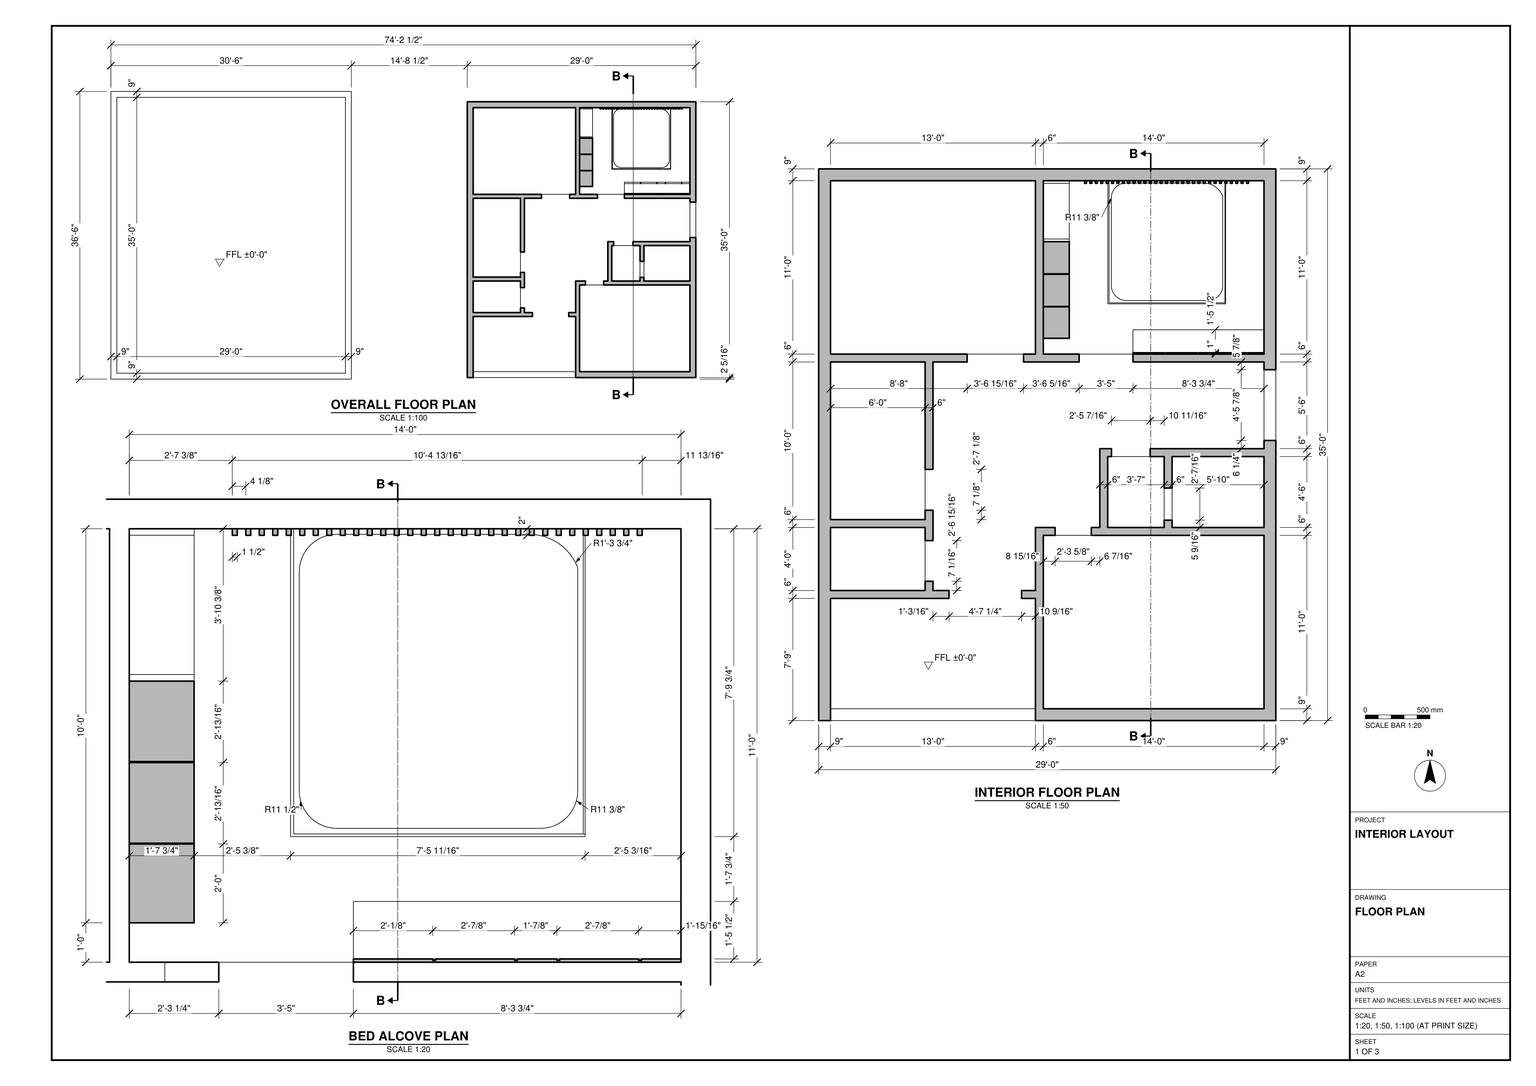
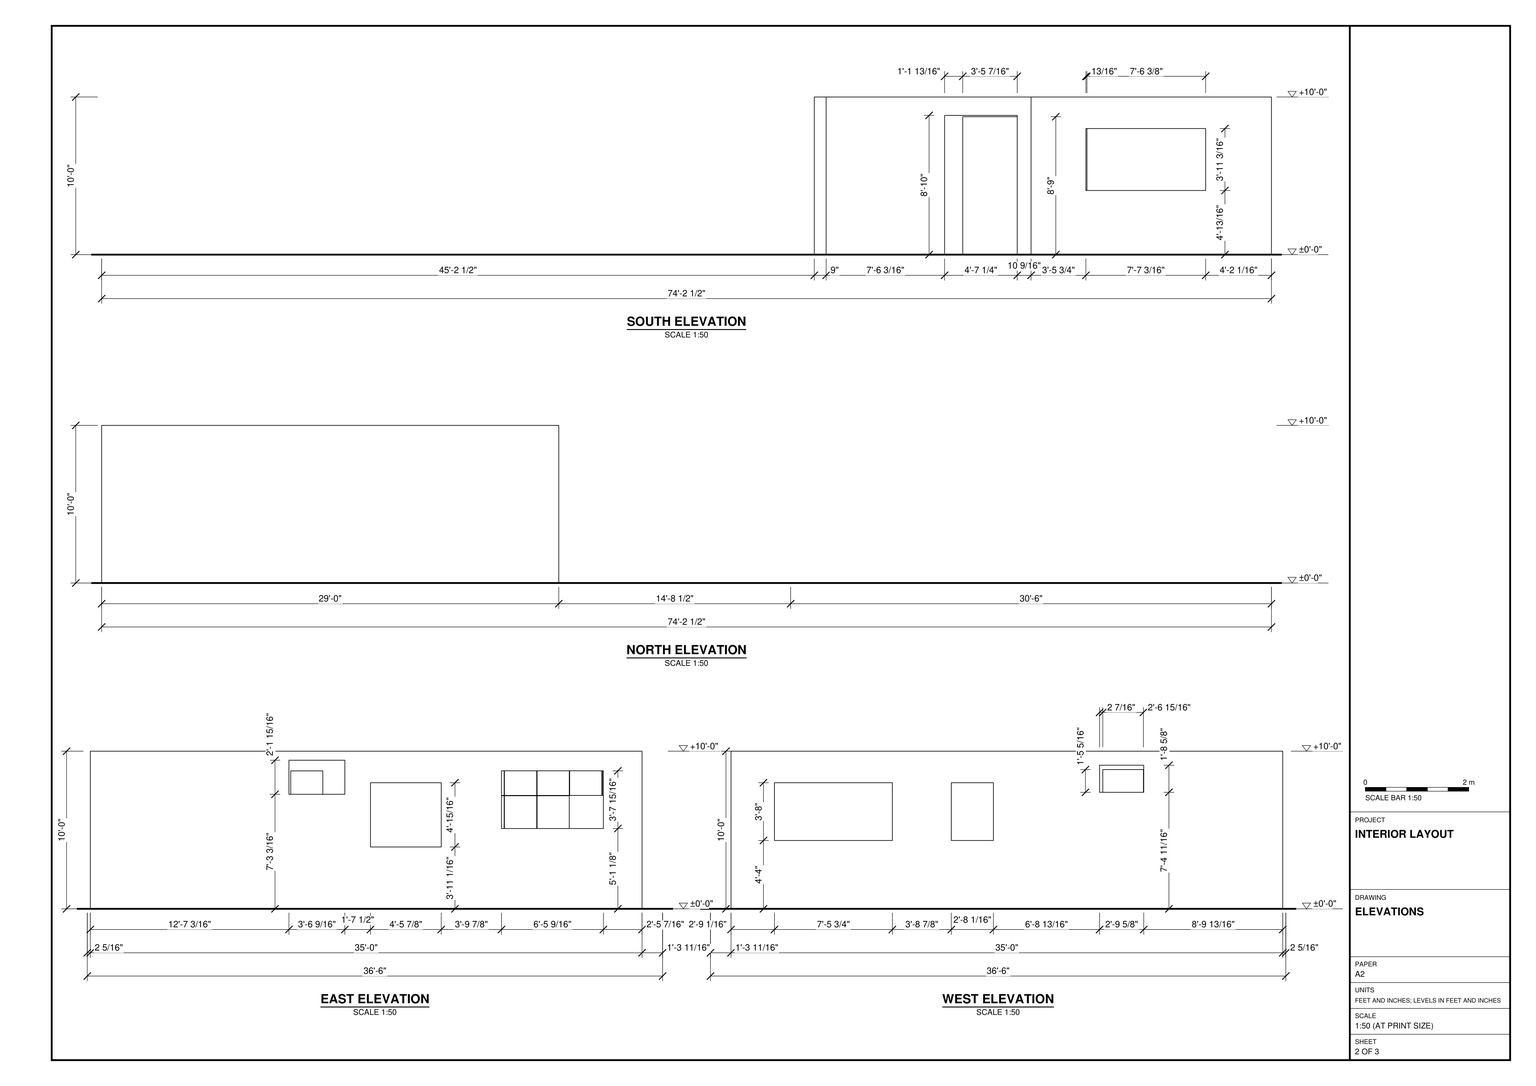
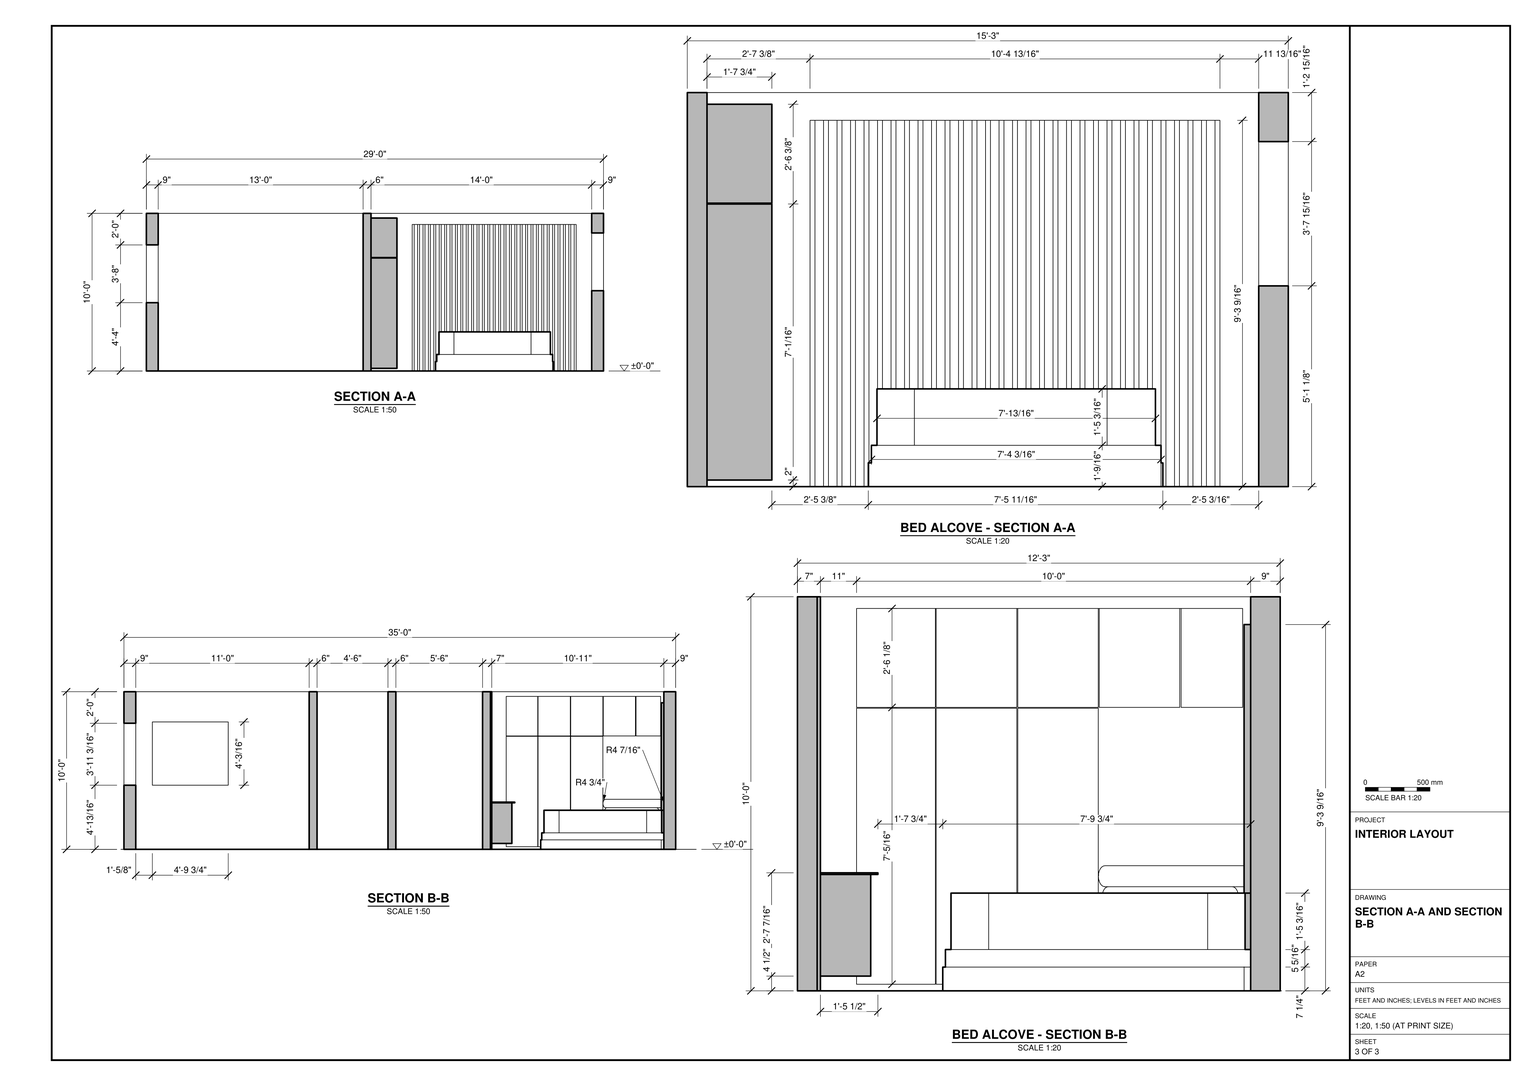
Work in feet and inches from task_files/diagram_01.pdf. Set the finished floor at ±0'-0". The full layout spans 74'-2 1/2" east to west, 36'-6" north to south and 10'-0" in height. Use the overall floor plan to place the flat, bordered rectangle on the west and the walled interior on the east. Leave the 14'-8 1/2" gap between them and follow the north and south offsets shown in plan.

Model the floor surfaces, exterior walls and partitions at their drawn thicknesses. Use the enlarged interior plan to set out the rooms and preserve the passages between them. Use the elevations to locate the south entrance and the window openings at their respective sill and head heights.

Fit out the northeast bed alcove using its enlarged plan and both sections. Model the stepped bed platform, the rounded mattress, the vertical slats behind the bed, the tall storage along the side wall and the shallow unit opposite the bed. Keep the entry beside the shallow unit clear. Make the shell elements and each furniture or joinery piece separate groups or components, and use components for repeated parts such as the slats. Any decor or loose items may be suitable library components. Save one SketchUp model as output_files/single_storey_interior_and_fitted_bed_alcove.skp.

# SketchUp Ruby script. Lengths in inches.
U = 1.inch
M = Sketchup.active_model
def pt(a) = Geom::Point3d.new(a.map { |v| v * U })
def face(e, loops, mat)
  f = e.add_face(loops[0].map { |a| pt(a) })
  loops[1..].each { |l| e.add_face(l.map { |a| pt(a) }).erase! }
  f.material = f.back_material = mat if mat
  f
end
# faces: each face lists its corners as indices into pts; further lists are holes
def faces(e, pts, list, mat = nil) = list.each { |f| face(e, (f[0].is_a?(Array) ? f : [f]).map { |l| l.map { |i| pts[i] } }, mat) }
# xy, xz, yz: faces in a plane at the given z, y or x. An outline is a flat list of corners, or four numbers for a rectangle; further outlines are holes
def ring(l) = l.size == 4 ? [[l[0], l[1]], [l[2], l[1]], [l[2], l[3]], [l[0], l[3]]] : l.each_slice(2).to_a
def flat(e, list, mat, &to3) = list.each { |f| face(e, (f[0].is_a?(Array) ? f : [f]).map { |l| ring(l).map { |u, v| to3.(u, v) } }, mat) }
def xy(e, z, list, mat = nil) = flat(e, list, mat) { |x, y| [x, y, z] }
def xz(e, y, list, mat = nil) = flat(e, list, mat) { |x, z| [x, y, z] }
def yz(e, x, list, mat = nil) = flat(e, list, mat) { |y, z| [x, y, z] }
def lines(e, pts, list) = list.each { |a, b| e.add_line(pt(pts[a]), pt(pts[b])) }
# prism: a flat outline (further loops are holes) pulled along v
def prism(e, loops, v, mat = nil)
  f = face(e, loops, mat); d = Geom::Vector3d.new(v.map { |x| x * U })
  f.pushpull(f.normal.samedirection?(d) ? d.length : -d.length)
end
def box(e, o, s, mat = nil) = prism(e, [[o, [o[0] + s[0], o[1], o[2]], [o[0] + s[0], o[1] + s[1], o[2]], [o[0], o[1] + s[1], o[2]]]], [0, 0, s[2]], mat)
def at(x, y, z, deg = 0) = Geom::Transformation.translation(pt([x, y, z])) * Geom::Transformation.rotation(ORIGIN, Z_AXIS, deg.degrees)
def axes(o, x, y, z) = Geom::Transformation.new([*x, 0, *y, 0, *z, 0, *pt(o).to_a, 1])
def part(name) = M.definitions.add(name)
# library, detail: a bought-in or finely detailed component or shape, given as its bounding box
def library(name, o, s) = part(name).tap { |d| box(d.entities, o, s) }
def detail(e, o, s) = box(e.add_group.entities, o, s)
def put(e, d, t, mat = nil) = e.add_instance(d, t).tap { |i| i.material = mat if mat }
def group(e, t, mat = nil) = e.add_group.tap { |g| g.transformation = t; g.material = mat if mat }.entities
root = M.entities
M.materials.add("[0099_LightSteelBlue]").color = [176, 196, 222]
M.materials.add("[Carrera Marble]").color = [207, 207, 207]
M.materials.add("[Color C07]").color = [153, 76, 0]
M.materials.add("[Color D06]").color = [204, 153, 0]
M.materials.add("[Suede Green]").color = [125, 126, 95]
M.materials.add("[Tile Canvas]").color = [199, 192, 173]
M.materials.add("[Wallpaper Thin Brown Stripes]").color = [182, 160, 118]
M.materials.add("[Wood Veneer 02]").color = [190, 128, 91]
xy(root,0,[[[0,0,366,438],[9,9,357,429]],[9,9,357,429],[551.52,11.34,707.52,11.34,707.52,95.34,699.55,95.34,699.55,101.34,707.52,101.34,707.52,149.34,722.48,149.34,722.48,143.34,750.09,143.34,750.09,149.34,756.52,149.34,756.52,209.34,765.4,209.34,765.4,203.34,794.85,203.34,794.85,209.34,881.52,209.34,881.52,275.34,781.77,275.34,781.77,281.34,724.34,281.34,724.34,275.34,698.46,275.34,698.46,281.34,655.52,281.34,655.52,275.34,629.52,275.34,629.52,193.59,623.52,193.59,623.52,162.46,629.52,162.46,629.52,139.34,623.52,139.34,623.52,108.4,629.52,108.4,629.52,101.34,641.71,101.34,641.71,95.34,551.52,95.34],[781.77,281.34,805.92,282.34],[805.92,281.34,806.82,281.9],
  [806.82,281.34,830.82,282.34],[830.82,281.34,831.72,281.9],[831.72,281.34,843.72,282.34],[843.72,281.34,844.625,281.9],[844.625,281.34,868.6,282.34],
  [868.6,281.34,869.53,281.9],[869.53,281.34,881.52,282.34],[744.9,411.34,746.4,413.34],[749.01,411.34,750.51,413.34],[753.12,411.34,754.62,413.34],
  [757.23,411.34,758.73,413.34],[855.88,411.34,857.38,413.34],[859.99,411.34,861.49,413.34],[864.1,411.34,865.6,413.34],[868.21,411.34,869.71,413.34]])
xy(root,0,[[762.65,319.59,762.65,411.34,762.84,411.34,762.84,413.34,851.77,413.34,851.77,411.34,852.33,411.34,852.33,319.59],[761.34,411.34,762.65,413.34],[762.65,411.34,762.84,413.34],[851.77,411.34,853.27,413.34]],"[Suede Green]")
xy(root,7.23,[[762.65,319.59,852.33,319.59,852.33,320.4,763.58,320.4,763.58,413.34,762.65,413.34],[851.77,320.4,852.33,411.34]],"[Suede Green]")
xy(root,12.57,[[[763.58,320.4,851.77,320.4,851.77,413.34,849.16,413.34,849.16,411.34,847.66,411.34,847.66,413.34,845.05,413.34,845.05,411.34,843.55,411.34,843.55,413.34,771.0625,413.34,771.0625,411.34,769.5625,411.34,769.5625,413.34,766.95,413.34,766.95,411.34,765.45,411.34,765.45,413.34,763.58,413.34],[776.75,322.1,775.25,322.2,773.78,322.49,772.36,322.97,771.02,323.63,769.77,324.47,768.64,325.46,767.65,326.59,766.82,327.83,766.15,329.18,765.67,330.6,765.38,332.07,765.28,333.57,765.28,400.26,765.375,401.74,765.67,403.2,766.15,404.61,766.8,405.95,767.63,407.1875,768.61,408.31,769.73,409.29,770.97,410.12,772.31,410.78,773.72,411.25,775.18,411.55,776.67,411.64,835.35,411.64,836.93,411.5625,838.5,411.32,840.03,410.93,841.52,410.38,842.94,409.69,844.29,408.86,845.55,407.89,846.7,406.81,847.74,405.61,848.66,404.31,849.4375,402.93,850.07,401.48,850.07,333.46,849.98,331.98,849.6875,330.52,849.21,329.11,848.55,327.78,847.73,326.54,846.75,325.43,845.63,324.45,844.39,323.62,843.06,322.96,841.65,322.48,840.19,322.19,838.71,322.1]]],"[Suede Green]")
xy(root,29.76,[[839.4375,411.34,840.9375,413.34]])
xy(root,29.76,[[776.75,322.1,838.71,322.1,840.19,322.19,841.65,322.48,843.06,322.96,844.39,323.62,845.63,324.45,846.75,325.43,847.73,326.54,848.55,327.78,849.21,329.11,849.6875,330.52,849.98,331.98,850.07,333.46,850.07,401.48,849.4375,402.93,848.66,404.31,847.74,405.61,846.7,406.81,845.55,407.89,844.29,408.86,842.94,409.69,841.52,410.38,840.03,410.93,838.5,411.32,836.93,411.5625,836.83,411.57,836.83,411.34,835.33,411.34,835.33,411.64,832.72,411.64,832.72,411.34,831.22,411.34,831.22,411.64,828.61,411.64,828.61,411.34,827.11,411.34,827.11,411.64,824.5,411.64,824.5,411.34,823,411.34,823,411.64,820.39,411.64,820.39,411.34,818.89,411.34,818.89,411.64,816.28,411.64,816.28,411.34,814.78,411.34,814.78,411.64,812.17,411.64,812.17,411.34,810.67,411.34,810.67,411.64,808.05,411.64,808.05,411.34,806.55,411.34,806.55,411.64,803.94,411.64,803.94,411.34,802.44,411.34,802.44,411.64,799.83,411.64,799.83,411.34,798.33,411.34,798.33,411.64,795.72,411.64,795.72,411.34,794.22,411.34,794.22,411.64,791.61,411.64,791.61,411.34,790.11,411.34,790.11,411.64,787.5,411.64,787.5,411.34,786,411.34,786,411.64,783.39,411.64,783.39,411.34,781.89,411.34,781.89,411.64,779.28,411.64,779.28,411.34,777.78,411.34,777.78,411.64,776.67,411.64,775.18,411.55,775.17,411.54,775.17,411.34,774.14,411.34,773.72,411.25,772.31,410.78,770.97,410.12,769.73,409.29,768.61,408.31,767.63,407.1875,766.8,405.95,766.15,404.61,765.67,403.2,765.375,401.74,765.28,400.26,765.28,333.57,765.38,332.07,765.67,330.6,766.15,329.18,766.82,327.83,767.65,326.59,768.64,325.46,769.77,324.47,771.02,323.63,772.36,322.97,773.78,322.49,775.25,322.2],[773.67,411.34,774.14,411.34,775.17,411.54,775.17,413.34,773.67,413.34],[774.14,411.34,775.17,411.34,775.17,411.54],[777.78,411.34,779.28,411.64],[781.89,411.34,783.39,411.64],
  [786,411.34,787.5,411.64],[790.11,411.34,791.61,411.64],[794.22,411.34,795.72,411.64],[798.33,411.34,799.83,411.64],[802.44,411.34,803.94,411.64],
  [806.55,411.34,808.05,411.64],[810.67,411.34,812.17,411.64],[814.78,411.34,816.28,411.64],[818.89,411.34,820.39,411.64],[823,411.34,824.5,411.64],
  [827.11,411.34,828.61,411.64],[831.22,411.34,832.72,411.64],[835.33,411.34,836.83,411.34,836.83,411.57,835.35,411.64,835.33,411.64],[836.83,411.57,836.83,413.34,835.33,413.34,835.33,411.64,835.35,411.64],[777.78,411.64,779.28,413.34],
  [781.89,411.64,783.39,413.34],[786,411.64,787.5,413.34],[790.11,411.64,791.61,413.34],[794.22,411.64,795.72,413.34],[798.33,411.64,799.83,413.34],
  [802.44,411.64,803.94,413.34],[806.55,411.64,808.05,413.34],[810.67,411.64,812.17,413.34],[814.78,411.64,816.28,413.34],[818.89,411.64,820.39,413.34],
  [823,411.64,824.5,413.34],[827.11,411.64,828.61,413.34],[831.22,411.64,832.72,413.34]],"[Suede Green]")
xy(root,111.55,[[744.9,411.34,746.4,413.34],[749.01,411.34,750.51,413.34],[753.12,411.34,754.62,413.34],[757.23,411.34,758.73,413.34],[761.34,411.34,762.84,413.34],
  [765.45,411.34,766.95,413.34],[769.5625,411.34,771.0625,413.34],[773.67,411.34,775.17,413.34],[777.78,411.34,779.28,413.34],[781.89,411.34,783.39,413.34],
  [786,411.34,787.5,413.34],[790.11,411.34,791.61,413.34],[794.22,411.34,795.72,413.34],[798.33,411.34,799.83,413.34],[802.44,411.34,803.94,413.34],
  [806.55,411.34,808.05,413.34],[810.67,411.34,812.17,413.34],[814.78,411.34,816.28,413.34],[818.89,411.34,820.39,413.34],[823,411.34,824.5,413.34],
  [827.11,411.34,828.61,413.34],[831.22,411.34,832.72,413.34],[835.33,411.34,836.83,413.34],[839.4375,411.34,840.9375,413.34],[843.55,411.34,845.05,413.34],
  [847.66,411.34,849.16,413.34],[851.77,411.34,853.27,413.34],[855.88,411.34,857.38,413.34],[859.99,411.34,861.49,413.34],[864.1,411.34,865.6,413.34],
  [868.21,411.34,869.71,413.34]],"[Wood Veneer 02]")
xy(root,120,[[805.92,281.34,806.82,281.9],[830.82,281.34,831.72,281.9],[843.72,281.34,844.625,281.9],[868.6,281.34,869.53,281.9]],"[Color D06]")
xy(root,120,[[781.77,281.34,805.92,282.34],[806.82,281.34,830.82,282.34],[831.72,281.34,843.72,282.34],[844.625,281.34,868.6,282.34],[869.53,281.34,881.52,282.34]],"[Wallpaper Thin Brown Stripes]")
xz(root,281.9,[[805.92,0,806.82,120],[830.82,0,831.72,120],[843.72,0,844.625,120],[868.6,0,869.53,120]],"[Color D06]")
xz(root,282.34,[[781.77,0,805.92,4.49],[806.82,0,830.82,4.49],[831.72,0,843.72,4.49],[844.625,0,868.6,4.49],[869.53,0,881.52,4.49],
  [781.77,4.49,805.92,35.4375],[805.92,4.49,806.82,35.4375],[806.82,4.49,830.82,35.4375],[830.82,4.49,831.72,35.4375],[831.72,4.49,843.72,35.4375],
  [843.72,4.49,844.625,35.4375],[844.625,4.49,868.6,35.4375],[868.6,4.49,869.53,35.4375]])
xz(root,282.34,[[781.77,35.4375,805.92,120],[806.82,35.4375,830.82,120],[831.72,35.4375,843.72,120],[844.625,35.4375,868.6,120],[869.53,35.4375,881.52,120]],"[Wallpaper Thin Brown Stripes]")
xz(root,319.59,[[762.65,0,852.33,7.23]],"[Suede Green]")
xz(root,320.4,[[763.58,7.23,851.77,12.57]],"[Suede Green]")
xz(root,322.1,[[776.75,12.57,838.71,29.76]],"[Suede Green]")
xz(root,411.34,[[851.77,0,852.33,7.23]],"[Suede Green]")
xz(root,411.34,[[744.9,0,746.4,111.55],[749.01,0,750.51,111.55],[753.12,0,754.62,111.55],[757.23,0,758.73,111.55],[761.34,0,762.84,111.55],
  [852.33,0,853.27,0,853.27,111.55,851.77,111.55,851.77,7.23,852.33,7.23],[855.88,0,857.38,111.55],[859.99,0,861.49,111.55],[864.1,0,865.6,111.55],[868.21,0,869.71,111.55],
  [765.45,12.57,766.95,111.55],[769.5625,12.57,771.0625,111.55],[843.55,12.57,845.05,111.55],[847.66,12.57,849.16,111.55],[773.67,29.76,775.17,111.55],
  [777.78,29.76,779.28,111.55],[781.89,29.76,783.39,111.55],[786,29.76,787.5,111.55],[790.11,29.76,791.61,111.55],[794.22,29.76,795.72,111.55],
  [798.33,29.76,799.83,111.55],[802.44,29.76,803.94,111.55],[806.55,29.76,808.05,111.55],[810.67,29.76,812.17,111.55],[814.78,29.76,816.28,111.55],
  [818.89,29.76,820.39,111.55],[823,29.76,824.5,111.55],[827.11,29.76,828.61,111.55],[831.22,29.76,832.72,111.55],[835.33,29.76,836.83,111.55],
  [839.4375,29.76,840.9375,111.55]],"[Wood Veneer 02]")
xz(root,411.64,[[776.67,12.57,835.35,29.76]],"[Suede Green]")
xz(root,413.34,[[744.9,0,746.4,37.01],[749.01,0,750.51,111.55],[753.12,0,754.62,111.55],[757.23,0,758.73,111.55],[855.88,0,857.38,111.55],
  [859.99,0,861.49,111.55],[864.1,0,865.6,111.55],[868.21,0,869.52,111.55],[869.52,0,869.71,37.01],[839.4375,29.76,840.9375,111.55]])
xz(root,413.34,[[761.34,0,762.65,0,762.65,7.23,762.84,7.23,762.84,111.55,761.34,111.55],[762.65,0,762.84,7.23],[762.84,0,762.84,7.23,763.58,7.23,763.58,12.57,765.45,12.57,765.45,27.14,766.95,27.14,766.95,12.57,769.5625,12.57,769.5625,27.14,771.0625,27.14,771.0625,12.57,843.55,12.57,843.55,27.14,845.05,27.14,845.05,12.57,847.66,12.57,847.66,27.14,849.16,27.14,849.16,12.57,851.77,12.57,851.77,0],[851.77,0,853.27,111.55],[765.45,27.14,766.95,111.55],
  [769.5625,27.14,771.0625,111.55],[843.55,27.14,845.05,111.55],[847.66,27.14,849.16,111.55],[773.67,29.76,775.17,111.55],[777.78,29.76,779.28,111.55],
  [781.89,29.76,783.39,111.55],[786,29.76,787.5,111.55],[790.11,29.76,791.61,111.55],[794.22,29.76,795.72,111.55],[798.33,29.76,799.83,111.55],
  [802.44,29.76,803.94,111.55],[806.55,29.76,808.05,111.55],[810.67,29.76,812.17,111.55],[814.78,29.76,816.28,111.55],[818.89,29.76,820.39,111.55],
  [823,29.76,824.5,111.55],[827.11,29.76,828.61,111.55],[831.22,29.76,832.72,111.55],[835.33,29.76,836.83,111.55]],"[Suede Green]")
yz(root,744.9,[[411.34,0,413.34,111.55]],"[Wood Veneer 02]")
yz(root,746.4,[[411.34,0,413.34,111.55]],"[Wood Veneer 02]")
yz(root,749.01,[[411.34,0,413.34,111.55]],"[Wood Veneer 02]")
yz(root,750.51,[[411.34,0,413.34,111.55]],"[Wood Veneer 02]")
yz(root,753.12,[[411.34,0,413.34,111.55]],"[Wood Veneer 02]")
yz(root,754.62,[[411.34,0,413.34,111.55]],"[Wood Veneer 02]")
yz(root,757.23,[[411.34,0,413.34,111.55]],"[Wood Veneer 02]")
yz(root,758.73,[[411.34,0,413.34,111.55]],"[Wood Veneer 02]")
yz(root,761.34,[[411.34,0,413.34,111.55]],"[Wood Veneer 02]")
yz(root,762.65,[[319.59,0,413.34,7.23]],"[Suede Green]")
yz(root,762.84,[[411.34,0,413.34,111.55]],"[Wood Veneer 02]")
yz(root,763.58,[[320.4,7.23,413.34,12.57]],"[Suede Green]")
yz(root,765.28,[[333.57,12.57,400.26,29.76]],"[Suede Green]")
yz(root,765.45,[[411.34,12.57,413.34,111.55]],"[Wood Veneer 02]")
yz(root,766.95,[[411.34,12.57,413.34,111.55]],"[Wood Veneer 02]")
yz(root,769.5625,[[411.34,12.57,413.34,111.55]],"[Wood Veneer 02]")
yz(root,771.0625,[[411.34,12.57,413.34,111.55]],"[Wood Veneer 02]")
yz(root,773.67,[[411.34,29.76,413.34,111.55]],"[Wood Veneer 02]")
yz(root,775.17,[[411.34,29.76,413.34,111.55]],"[Wood Veneer 02]")
yz(root,777.78,[[411.34,29.76,413.34,111.55]],"[Wood Veneer 02]")
yz(root,779.28,[[411.34,29.76,413.34,111.55]],"[Wood Veneer 02]")
yz(root,781.77,[[281.34,0,282.34,120]],"[Color D06]")
yz(root,781.89,[[411.34,29.76,413.34,111.55]],"[Wood Veneer 02]")
yz(root,783.39,[[411.34,29.76,413.34,111.55]],"[Wood Veneer 02]")
yz(root,786,[[411.34,29.76,413.34,111.55]],"[Wood Veneer 02]")
yz(root,787.5,[[411.34,29.76,413.34,111.55]],"[Wood Veneer 02]")
yz(root,790.11,[[411.34,29.76,413.34,111.55]],"[Wood Veneer 02]")
yz(root,791.61,[[411.34,29.76,413.34,111.55]],"[Wood Veneer 02]")
yz(root,794.22,[[411.34,29.76,413.34,111.55]],"[Wood Veneer 02]")
yz(root,795.72,[[411.34,29.76,413.34,111.55]],"[Wood Veneer 02]")
yz(root,798.33,[[411.34,29.76,413.34,111.55]],"[Wood Veneer 02]")
yz(root,799.83,[[411.34,29.76,413.34,111.55]],"[Wood Veneer 02]")
yz(root,802.44,[[411.34,29.76,413.34,111.55]],"[Wood Veneer 02]")
yz(root,803.94,[[411.34,29.76,413.34,111.55]],"[Wood Veneer 02]")
yz(root,805.92,[[297.15,4.49,297.65,35.4375]])
yz(root,805.92,[[281.9,0,282.34,120]],"[Color D06]")
yz(root,806.55,[[411.34,29.76,413.34,111.55]],"[Wood Veneer 02]")
yz(root,806.82,[[281.9,0,282.34,120],[297.15,4.49,297.65,35.4375]],"[Color D06]")
yz(root,808.05,[[411.34,29.76,413.34,111.55]],"[Wood Veneer 02]")
yz(root,810.67,[[411.34,29.76,413.34,111.55]],"[Wood Veneer 02]")
yz(root,812.17,[[411.34,29.76,413.34,111.55]],"[Wood Veneer 02]")
yz(root,814.78,[[411.34,29.76,413.34,111.55]],"[Wood Veneer 02]")
yz(root,816.28,[[411.34,29.76,413.34,111.55]],"[Wood Veneer 02]")
yz(root,818.89,[[411.34,29.76,413.34,111.55]],"[Wood Veneer 02]")
yz(root,820.39,[[411.34,29.76,413.34,111.55]],"[Wood Veneer 02]")
yz(root,823,[[411.34,29.76,413.34,111.55]],"[Wood Veneer 02]")
yz(root,824.5,[[411.34,29.76,413.34,111.55]],"[Wood Veneer 02]")
yz(root,827.11,[[411.34,29.76,413.34,111.55]],"[Wood Veneer 02]")
yz(root,828.61,[[411.34,29.76,413.34,111.55]],"[Wood Veneer 02]")
yz(root,830.82,[[281.9,0,282.34,120]],"[Color D06]")
yz(root,831.22,[[411.34,29.76,413.34,111.55]],"[Wood Veneer 02]")
yz(root,831.72,[[281.9,0,282.34,120],[297.15,4.49,297.65,35.4375]],"[Color D06]")
yz(root,832.72,[[411.34,29.76,413.34,111.55]],"[Wood Veneer 02]")
yz(root,835.33,[[411.34,29.76,413.34,111.55]],"[Wood Veneer 02]")
yz(root,836.83,[[411.34,29.76,413.34,111.55]],"[Wood Veneer 02]")
yz(root,839.4375,[[411.34,29.76,413.34,111.55]],"[Wood Veneer 02]")
yz(root,840.9375,[[411.34,29.76,413.34,111.55]],"[Wood Veneer 02]")
yz(root,843.55,[[411.34,12.57,413.34,111.55]],"[Wood Veneer 02]")
yz(root,843.72,[[297.15,4.49,297.65,35.4375]])
yz(root,843.72,[[281.9,0,282.34,120]],"[Color D06]")
yz(root,844.625,[[281.9,0,282.34,120],[297.15,4.49,297.65,35.4375]],"[Color D06]")
yz(root,845.05,[[411.34,12.57,413.34,111.55]],"[Wood Veneer 02]")
yz(root,847.66,[[411.34,12.57,413.34,111.55]],"[Wood Veneer 02]")
yz(root,849.16,[[411.34,12.57,413.34,111.55]],"[Wood Veneer 02]")
yz(root,850.07,[[333.46,12.57,401.48,29.76]],"[Suede Green]")
yz(root,851.77,[[411.34,0,413.34,12.57],[320.4,7.23,411.34,12.57]],"[Suede Green]")
yz(root,851.77,[[411.34,12.57,413.34,111.55]],"[Wood Veneer 02]")
yz(root,852.33,[[319.59,0,411.34,7.23]],"[Suede Green]")
yz(root,853.27,[[411.34,0,413.34,111.55]],"[Wood Veneer 02]")
yz(root,855.88,[[411.34,0,413.34,111.55]],"[Wood Veneer 02]")
yz(root,857.38,[[411.34,0,413.34,111.55]],"[Wood Veneer 02]")
yz(root,859.99,[[411.34,0,413.34,111.55]],"[Wood Veneer 02]")
yz(root,861.49,[[411.34,0,413.34,111.55]],"[Wood Veneer 02]")
yz(root,864.1,[[411.34,0,413.34,111.55]],"[Wood Veneer 02]")
yz(root,865.6,[[411.34,0,413.34,111.55]],"[Wood Veneer 02]")
yz(root,868.21,[[411.34,0,413.34,111.55]],"[Wood Veneer 02]")
yz(root,868.6,[[281.9,0,282.34,120]],"[Color D06]")
yz(root,869.53,[[281.9,0,282.34,120],[297.15,4.49,297.65,35.4375]],"[Color D06]")
yz(root,869.71,[[411.34,0,413.34,111.55]],"[Wood Veneer 02]")
yz(root,881.52,[[281.34,0,282.34,0,282.34,4.49,297.65,4.49,297.65,35.4375,282.34,35.4375,282.34,120,281.34,120]])
p = [[775.25,322.2,29.76],[775.25,322.2,12.57],[776.75,322.1,12.57],[776.75,322.1,29.76],[838.71,322.1,29.76],[838.71,322.1,12.57],
  [840.19,322.19,12.57],[840.19,322.19,29.76],[773.78,322.49,29.76],[773.78,322.49,12.57],[841.65,322.48,12.57],[841.65,322.48,29.76],
  [772.36,322.97,29.76],[772.36,322.97,12.57],[843.06,322.96,12.57],[843.06,322.96,29.76],[771.02,323.63,29.76],[771.02,323.63,12.57],
  [844.39,323.62,12.57],[844.39,323.62,29.76],[769.77,324.47,29.76],[769.77,324.47,12.57],[845.63,324.45,12.57],[845.63,324.45,29.76],
  [846.75,325.43,12.57],[846.75,325.43,29.76],[768.64,325.46,29.76],[768.64,325.46,12.57],[847.73,326.54,12.57],[847.73,326.54,29.76],
  [767.65,326.59,29.76],[767.65,326.59,12.57],[848.55,327.78,12.57],[848.55,327.78,29.76],[766.82,327.83,29.76],[766.82,327.83,12.57],
  [766.15,329.18,29.76],[766.15,329.18,12.57],[849.21,329.11,12.57],[849.21,329.11,29.76],[849.6875,330.52,12.57],[849.6875,330.52,29.76],
  [765.67,330.6,29.76],[765.67,330.6,12.57],[849.98,331.98,12.57],[849.98,331.98,29.76],[765.38,332.07,29.76],[765.38,332.07,12.57],
  [850.07,333.46,12.57],[850.07,333.46,29.76],[765.28,333.57,29.76],[765.28,333.57,12.57],[765.375,401.74,29.76],[765.375,401.74,12.57],
  [765.28,400.26,12.57],[765.28,400.26,29.76],[850.07,401.48,29.76],[850.07,401.48,12.57],[849.4375,402.93,12.57],[849.4375,402.93,29.76],
  [765.67,403.2,29.76],[765.67,403.2,12.57],[848.66,404.31,12.57],[848.66,404.31,29.76],[766.15,404.61,29.76],[766.15,404.61,12.57],
  [847.74,405.61,12.57],[847.74,405.61,29.76],[766.8,405.95,29.76],[766.8,405.95,12.57],[846.7,406.81,12.57],[846.7,406.81,29.76],
  [767.63,407.1875,29.76],[767.63,407.1875,12.57],[845.55,407.89,12.57],[845.55,407.89,29.76],[768.61,408.31,29.76],[768.61,408.31,12.57],
  [844.29,408.86,12.57],[844.29,408.86,29.76],[769.73,409.29,29.76],[769.73,409.29,12.57],[842.94,409.69,12.57],[842.94,409.69,29.76],
  [770.97,410.12,29.76],[770.97,410.12,12.57],[841.52,410.38,12.57],[841.52,410.38,29.76],[772.31,410.78,29.76],[772.31,410.78,12.57],
  [840.03,410.93,12.57],[840.03,410.93,29.76],[773.72,411.25,29.76],[773.72,411.25,12.57],[838.5,411.32,12.57],[838.5,411.32,29.76],
  [775.18,411.55,29.76],[775.18,411.55,12.57],[774.14,411.34,29.76],[775.17,411.54,29.76],[836.93,411.5625,12.57],[836.93,411.5625,29.76],
  [776.67,411.64,29.76],[776.67,411.64,12.57],[835.35,411.64,12.57],[835.35,411.64,29.76],[836.83,411.57,29.76],[781.77,297.65,35.4375],
  [805.92,297.65,35.4375],[806.82,297.65,35.4375],[831.72,297.65,35.4375],[843.72,297.65,35.4375],[844.625,297.65,35.4375],[869.53,297.65,35.4375],
  [881.52,297.65,35.4375],[746.4,413.34,111.55],[749.01,413.34,111.55],[750.51,413.34,111.55],[753.12,413.34,111.55],[754.62,413.34,111.55],
  [757.23,413.34,111.55],[758.73,413.34,111.55],[761.34,413.34,111.55],[762.84,413.34,111.55],[765.45,413.34,111.55],[766.95,413.34,111.55],
  [769.5625,413.34,111.55],[771.0625,413.34,111.55],[773.67,413.34,111.55],[775.17,413.34,111.55],[777.78,413.34,111.55],[779.28,413.34,111.55],
  [781.89,413.34,111.55],[783.39,413.34,111.55],[786,413.34,111.55],[787.5,413.34,111.55],[790.11,413.34,111.55],[791.61,413.34,111.55],
  [794.22,413.34,111.55],[795.72,413.34,111.55],[798.33,413.34,111.55],[799.83,413.34,111.55],[802.44,413.34,111.55],[803.94,413.34,111.55],
  [806.55,413.34,111.55],[808.05,413.34,111.55],[810.67,413.34,111.55],[812.17,413.34,111.55],[814.78,413.34,111.55],[816.28,413.34,111.55],
  [818.89,413.34,111.55],[820.39,413.34,111.55],[823,413.34,111.55],[824.5,413.34,111.55],[827.11,413.34,111.55],[828.61,413.34,111.55],
  [831.22,413.34,111.55],[832.72,413.34,111.55],[835.33,413.34,111.55],[836.83,413.34,111.55],[839.4375,413.34,111.55],[840.9375,413.34,111.55],
  [843.55,413.34,111.55],[845.05,413.34,111.55],[847.66,413.34,111.55],[849.16,413.34,111.55],[851.77,413.34,111.55],[853.27,413.34,111.55],
  [855.88,413.34,111.55],[857.38,413.34,111.55],[859.99,413.34,111.55],[861.49,413.34,111.55],[864.1,413.34,111.55],[865.6,413.34,111.55],
  [868.21,413.34,111.55],[781.77,282.34,35.4375]]
faces(root,p,[[0,1,2,3],[4,5,6,7],[8,9,1,0],[7,6,10,11],[12,13,9,8],[11,10,14,15],[16,17,13,12],[15,14,18,19],
  [20,21,17,16],[19,18,22,23],[23,22,24,25],[26,27,21,20],[25,24,28,29],[30,31,27,26],[29,28,32,33],[34,35,31,30],
  [36,37,35,34],[33,32,38,39],[39,38,40,41],[42,43,37,36],[41,40,44,45],[46,47,43,42],[45,44,48,49],[50,51,47,46],
  [52,53,54,55],[56,57,58,59],[60,61,53,52],[59,58,62,63],[64,65,61,60],[63,62,66,67],[68,69,65,64],[67,66,70,71],
  [72,73,69,68],[71,70,74,75],[76,77,73,72],[75,74,78,79],[80,81,77,76],[79,78,82,83],[84,85,81,80],[83,82,86,87],
  [88,89,85,84],[87,86,90,91],[92,93,89,88],[91,90,94,95],[96,97,93,92,98,99],[95,94,100,101],[102,103,97,96],[101,100,104,105,106]],"[Suede Green]")
lines(root,p,[[107,108],[109,110],[108,109],[110,111],[112,113],[111,112],[113,114],[115,116],[117,118],[119,120],[121,122],[123,124],
  [125,126],[127,128],[129,130],[131,132],[133,134],[135,136],[137,138],[139,140],[141,142],[143,144],[145,146],[147,148],
  [149,150],[151,152],[153,154],[155,156],[157,158],[159,160],[161,162],[163,164],[165,166],[167,168],[169,170],[171,172],
  [173,174],[107,175]])
g1 = group(root,at(551.52,281.34,0))
xy(g1,0,[[0,0,156,132]])
g2 = group(root,at(713.52,281.34,0))
xy(g2,0,[[0,0,168,132]],"[Tile Canvas]")
g3 = group(root,at(551.52,155.34,0))
xy(g3,0,[[0,0,72,120]])
g4 = group(root,at(551.52,101.34,0))
xy(g4,0,[[0,0,72,48]])
g5 = group(root,at(762.52,149.34,0))
xy(g5,0,[[0,0,43,54]])
g6 = group(root,at(811.52,149.34,0))
xy(g6,0,[[0,0,70,54]])
g7 = group(root,at(713.52,11.34,0))
xy(g7,0,[[0,0,168,132]])
g8 = group(root,at(713.52,281.34,0))
xy(g8,2,[[0,12,19.75,36],[0,36.24,19.75,60.8],[0,61.1,19.75,85.6]])
xy(g8,25.88,[[3.375,88.72,18.84,126.44]],"[Carrera Marble]")
xy(g8,31.7,[[0,87.61,0,130.03,19.75,130.03,19.75,129.78,3.375,129.78,3.375,87.61],[3.375,87.61,19.75,88.72],[18.84,88.72,19.75,126.43],[3.375,126.43,19.75,129.78]])
xy(g8,38.1,[[0,87.61,19.75,130.03]],"[Carrera Marble]")
xy(g8,86.0625,[[0,12,19.75,36],[0,36.24,19.75,60.8],[0,61.1,19.75,85.6]],"[Wood Veneer 02]")
xy(g8,86.3125,[[0,12,19.75,36],[0,36.24,19.75,60.8],[0,61.1,19.75,85.6],[0,85.9,19.75,110.4],[0,110.83,19.75,129.5625]])
xy(g8,116.4375,[[0,12,19.75,36],[0,36.24,19.75,60.8],[0,61.1,19.75,85.6],[0,85.9,19.75,110.4],[0,110.83,19.75,129.5625]],"[Color C07]")
xz(g8,12,[[0,86.3125,19.75,116.4375]],"[Color C07]")
xz(g8,12,[[0,2,19.75,86.0625]],"[Wood Veneer 02]")
xz(g8,36,[[0,86.3125,19.75,116.4375]],"[Color C07]")
xz(g8,36,[[0,2,19.75,86.0625]],"[Wood Veneer 02]")
xz(g8,36.24,[[0,86.3125,19.75,116.4375]],"[Color C07]")
xz(g8,36.24,[[0,2,19.75,86.0625]],"[Wood Veneer 02]")
xz(g8,60.8,[[0,86.3125,19.75,116.4375]],"[Color C07]")
xz(g8,60.8,[[0,2,19.75,86.0625]],"[Wood Veneer 02]")
xz(g8,61.1,[[0,86.3125,19.75,116.4375]],"[Color C07]")
xz(g8,61.1,[[0,2,19.75,86.0625]],"[Wood Veneer 02]")
xz(g8,85.6,[[0,2,19.75,36.47]])
xz(g8,85.6,[[0,86.3125,19.75,116.4375]],"[Color C07]")
xz(g8,85.6,[[0,36.47,19.75,86.0625]],"[Wood Veneer 02]")
xz(g8,85.9,[[0,86.3125,19.75,116.4375]],"[Color C07]")
xz(g8,110.4,[[0,86.3125,19.75,116.4375]],"[Color C07]")
xz(g8,110.83,[[0,86.3125,19.75,116.4375]],"[Color C07]")
xz(g8,129.5625,[[0,86.3125,19.75,116.4375]])
yz(g8,0,[[87.61,31.7,130.03,31.7,131.74,33.32,131.9375,35.69,131.93,35.73,131.74,36.5,131.46,37.08,130.03,38.1,87.61,38.1,86.19,37.11,85.9,36.5,85.71,35.73,85.6875,35.52,85.89,33.33,85.92,33.27],[87.61,31.7,85.92,33.27,86.22,32.64,86.625,32.13,87.1,31.81],[130.03,31.7,130.54,31.81,131.01,32.13,131.42,32.64,131.74,33.3,131.74,33.32],[131.74,33.32,131.93,34.07,132,34.9,131.9375,35.69],[85.89,33.33,85.6875,35.52,85.64,34.9,85.71,34.07],
  [132,34.9,132,36.47,131.9375,35.69],[131.46,37.08,131.42,37.17,131.01,37.67,130.54,37.99,130.03,38.1],[86.19,37.11,87.61,38.1,87.1,37.99,86.625,37.67,86.22,37.17]])
yz(g8,3.375,[[88.72,25.88,88.24,25.95,87.78,26.22,87.39,26.67,87.08,27.29,86.89,28.01,86.82,28.79,86.89,29.57,87.08,30.3,87.39,30.91,87.78,31.37,88.24,31.64,88.72,31.7,126.43,31.7,126.9,31.6,127.33,31.3125,127.7,30.85,127.99,30.25,128.17,29.55,128.23,28.8,128.17,28.05,127.99,27.34,127.71,26.74,127.34,26.28,126.91,25.99,126.44,25.88]])
yz(g8,18.84,[[88.72,25.88,126.44,25.88,126.91,25.99,127.34,26.28,127.71,26.74,127.99,27.34,128.17,28.05,128.23,28.8,128.17,29.55,127.99,30.25,127.7,30.85,127.33,31.3125,126.9,31.6,126.43,31.7,88.72,31.7,88.24,31.64,87.78,31.37,87.39,30.91,87.08,30.3,86.89,29.57,86.82,28.79,86.89,28.01,87.08,27.29,87.39,26.67,87.78,26.22,88.24,25.95]],"[Carrera Marble]")
yz(g8,19.75,[[87.61,31.7,130.03,31.7,130.54,31.81,131.01,32.13,131.42,32.64,131.74,33.3,131.93,34.07,132,34.9,131.93,35.73,131.74,36.5,131.42,37.17,131.01,37.67,130.54,37.99,130.03,38.1,87.61,38.1,87.1,37.99,86.625,37.67,86.22,37.17,85.9,36.5,85.71,35.73,85.64,34.9,85.71,34.07,85.9,33.3,86.22,32.64,86.625,32.13,87.1,31.81]],"[Carrera Marble]")
yz(g8,19.75,[[12,86.3125,36,116.4375],[36.24,86.3125,60.8,116.4375],[61.1,86.3125,85.6,116.4375],[85.9,86.3125,110.4,116.4375],[110.83,86.3125,129.5625,116.4375]],"[Color C07]")
yz(g8,19.75,[[12,2,36,86.0625],[36.24,2,60.8,86.0625],[61.1,2,85.6,86.0625]],"[Wood Veneer 02]")
p = [[18.84,88.24,25.95],[18.84,87.78,26.22],[3.375,87.78,26.22],[3.375,88.24,25.95],[18.84,88.72,25.88],[3.375,88.72,25.88],
  [18.84,126.91,25.99],[18.84,126.44,25.88],[3.375,126.44,25.88],[3.375,126.91,25.99],[18.84,127.34,26.28],[3.375,127.34,26.28],
  [18.84,87.39,26.67],[3.375,87.39,26.67],[18.84,127.71,26.74],[3.375,127.71,26.74],[18.84,87.08,27.29],[3.375,87.08,27.29],
  [18.84,127.99,27.34],[3.375,127.99,27.34],[18.84,86.89,28.01],[3.375,86.89,28.01],[18.84,128.17,28.05],[3.375,128.17,28.05],
  [18.84,86.82,28.79],[3.375,86.82,28.79],[18.84,128.23,28.8],[3.375,128.23,28.8],[18.84,86.89,29.57],[3.375,86.89,29.57],
  [18.84,128.17,29.55],[3.375,128.17,29.55],[18.84,87.08,30.3],[3.375,87.08,30.3],[18.84,127.99,30.25],[3.375,127.99,30.25],
  [18.84,87.39,30.91],[3.375,87.39,30.91],[18.84,127.7,30.85],[3.375,127.7,30.85],[18.84,87.78,31.37],[3.375,87.78,31.37],
  [18.84,127.33,31.3125],[3.375,127.33,31.3125],[18.84,126.9,31.6],[3.375,126.9,31.6],[18.84,88.24,31.64],[3.375,88.24,31.64],
  [18.84,88.72,31.7],[3.375,88.72,31.7],[18.84,126.43,31.7],[3.375,126.43,31.7],[19.75,87.61,31.7],[19.75,87.1,31.81],
  [0,87.1,31.81],[0,87.61,31.7],[3.375,87.61,31.7],[19.75,130.54,31.81],[19.75,130.03,31.7],[0,130.03,31.7],
  [0,130.54,31.81],[19.75,86.625,32.13],[0,86.625,32.13],[19.75,131.01,32.13],[0,131.01,32.13],[19.75,86.22,32.64],
  [0,86.22,32.64],[19.75,131.42,32.64],[0,131.42,32.64],[19.75,85.9,33.3],[0,85.9,33.3],[0,85.92,33.27],
  [19.75,131.74,33.3],[0,131.74,33.3],[19.75,85.71,34.07],[0,85.71,34.07],[0,85.89,33.33],[19.75,131.93,34.07],
  [0,131.74,33.32],[0,131.93,34.07],[19.75,85.64,34.9],[0,85.64,34.9],[19.75,132,34.9],[0,132,34.9],
  [19.75,85.71,35.73],[0,85.71,35.73],[0,85.6875,35.52],[19.75,131.93,35.73],[0,131.9375,35.69],[0,131.93,35.73],
  [19.75,85.9,36.5],[0,85.9,36.5],[19.75,131.74,36.5],[0,131.74,36.5],[19.75,86.22,37.17],[0,86.22,37.17],
  [0,86.19,37.11],[19.75,131.42,37.17],[0,131.46,37.08],[0,131.42,37.17],[19.75,86.625,37.67],[0,86.625,37.67],
  [19.75,131.01,37.67],[0,131.01,37.67],[19.75,87.1,37.99],[0,87.1,37.99],[19.75,130.54,37.99],[0,130.54,37.99],
  [19.75,87.61,38.1],[0,87.61,38.1],[19.75,130.03,38.1],[0,130.03,38.1],[0,0,0],[0,132,0],
  [0,132,120],[0,0,120],[0,36.24,116.4375],[0,36,116.4375],[0,61.1,116.4375],[0,60.8,116.4375],
  [0,85.9,116.4375],[0,85.6,116.4375],[0,110.83,116.4375],[0,110.4,116.4375],[0,85.6,36.47],[0,132,36.47]]
faces(g8,p,[[0,1,2,3],[4,0,3,5],[1,12,13,2],[12,16,17,13],[16,20,21,17],[20,24,25,21],[24,28,29,25],[28,32,33,29],
  [32,36,37,33],[36,40,41,37],[40,46,47,41],[46,48,49,47],[52,53,54,55,56],[57,58,59,60],[53,61,62,54],[63,57,60,64],
  [61,65,66,62],[67,63,64,68],[65,69,70,71,66],[72,67,68,73],[69,74,75,76,70],[77,72,73,78,79],[74,80,81,75],[82,77,79,83],
  [80,84,85,86,81],[87,82,83,88,89],[84,90,91,85],[92,87,89,93],[90,94,95,96,91],[97,92,93,98,99],[94,100,101,95],[102,97,99,103],
  [100,104,105,101],[106,102,103,107],[104,108,109,105],[110,106,107,111]],"[Carrera Marble]")
faces(g8,p,[[6,7,8,9],[10,6,9,11],[14,10,11,15],[18,14,15,19],[22,18,19,23],[26,22,23,27],[30,26,27,31],[34,30,31,35],
  [38,34,35,39],[42,38,39,43],[44,42,43,45],[50,44,45,51]])
lines(g8,p,[[112,113],[113,83],[114,115],[115,112],[116,117],[118,119],[120,121],[122,123],[124,86],[125,114]])
g9 = group(root,at(781.77,282.34,4.49))
xy(g9,0,[[0,0,24.15,15.3125],[24.15,0,25.05,14.8125],[25.05,0,49.05,15.3125],[49.05,0,49.95,14.8125],[49.95,0,61.95,15.3125],
  [61.95,0,62.85,14.8125],[62.85,0,86.83,15.3125],[86.83,0,87.76,14.8125],[87.76,0,99.75,15.3125]])
xy(g9,30.95,[[0,0,0,15.3125,24.15,15.3125,24.15,14.8125,25.05,14.8125,25.05,15.3125,49.05,15.3125,49.05,14.8125,49.95,14.8125,49.95,15.3125,61.95,15.3125,61.95,14.8125,62.85,14.8125,62.85,15.3125,86.83,15.3125,86.83,14.8125,87.76,14.8125,87.76,15.3125,99.75,15.3125,99.75,0],[24.15,14.8125,25.05,17.5],[49.05,14.8125,49.95,17.5],[61.95,14.8125,62.85,17.5],[86.83,14.8125,87.76,17.5],
  [0,15.3125,24.15,17.5],[25.05,15.3125,49.05,17.5],[49.95,15.3125,61.95,17.5],[62.85,15.3125,86.83,17.5],[87.76,15.3125,99.75,17.5]])
xy(g9,31.45,[[0,0,99.75,17.5]],"[Carrera Marble]")
xz(g9,0,[[0,30.95,24.15,31.45],[24.15,30.95,25.05,31.45],[25.05,30.95,49.05,31.45],[49.05,30.95,49.95,31.45],[49.95,30.95,61.95,31.45],
  [61.95,30.95,62.85,31.45],[62.85,30.95,86.83,31.45],[86.83,30.95,87.76,31.45],[87.76,30.95,99.75,31.45]])
xz(g9,14.8125,[[24.15,0,25.05,30.95],[49.05,0,49.95,30.95],[61.95,0,62.85,30.95],[86.83,0,87.76,30.95]],"[Color D06]")
xz(g9,15.3125,[[0,0,24.15,30.95],[25.05,0,49.05,30.95],[49.95,0,61.95,30.95],[62.85,0,86.83,30.95],[87.76,0,99.75,30.95]],"[Wallpaper Thin Brown Stripes]")
xz(g9,17.5,[[0,30.95,99.75,31.45]],"[Carrera Marble]")
yz(g9,0,[[0,30.95,17.5,31.45]],"[Carrera Marble]")
yz(g9,0,[[0,0,15.3125,30.95]],"[Wallpaper Thin Brown Stripes]")
yz(g9,49.05,[[14.8125,0,15.3125,30.95]],"[Color D06]")
yz(g9,86.83,[[14.8125,0,15.3125,30.95]],"[Color D06]")
yz(g9,99.75,[[0,30.95,17.5,31.45]])
g10 = group(root,at(542.52,2.34,0))
xy(g10,0,[[0,0,0,420,348,420,348,0,165,0,165,93,154.46,93,154.46,99,165,99,165,147,179.95,147,179.95,141,171,141,171,9,339,9,339,141,207.5625,141,207.5625,147,214,147,214,207,222.875,207,222.875,201,220,201,220,147,263,147,263,152.5625,269,152.5625,269,147,339,147,339,201,269,201,269,177,263,177,263,201,252.33,201,252.33,207,339,207,339,273,239.25,273,239.25,279,339,279,339,411,171,411,171,279,198.25,279,198.25,273,155.9375,273,155.9375,279,165,279,165,411,9,411,9,279,113,279,113,273,87,273,87,191.25,81,191.25,81,273,9,273,9,153,81,153,81,160.125,87,160.125,87,137,81,137,81,147,9,147,9,99,81,99,81,106.0625,87,106.0625,87,99,99.1875,99,99.1875,93,9,93,9,0],[9,0,165,9],[263,152.5625,269,177]])
xy(g10,47.0625,[[339,213.25,348,267.125]])
xy(g10,48.8125,[[206.75,0,297.9375,9],[165,21.625,171,79.375]])
xy(g10,52,[[0,220.26,9,252.3125],[0,297.1875,9,386.9375]])
xy(g10,61.125,[[339,313,348,390.5625]])
xy(g10,87.1875,[[339,151.1875,348,193.75]])
xy(g10,88.6875,[[0,105.8125,9,139.4375]])
xy(g10,96,[[206.75,0,297.9375,9],[339,213.25,348,267.125],[0,220.26,9,252.3125],[0,297.1875,9,386.9375]])
xy(g10,97,[[165,21.625,171,79.375]])
xy(g10,105,[[179.95,141,207.5625,147],[263,152.5625,269,177],[222.875,201,252.33,207],[113,273,155.9375,279],[198.25,273,239.25,279]])
xy(g10,105.0625,[[339,313,348,390.5625]])
xy(g10,106,[[99.1875,93,154.46,99],[81,106.0625,87,137],[81,160.125,87,191.25]])
xy(g10,109.3125,[[0,105.8125,9,139.4375]])
xy(g10,113.125,[[339,151.1875,348,193.75]])
xy(g10,120,[[[0,0,9,0,9,93,165,93,165,0,348,0,348,420,0,420],[87,99,87,273,339,273,339,207,214,207,214,147,165,147,165,99],[171,279,339,411],[171,9,339,141],[9,279,165,411],[9,153,81,273],[269,147,339,201],[9,99,81,147],[220,147,263,201]]])
xz(g10,0,[[0,0,9,120],[[165,0,348,120],[206.75,48.8125,297.9375,96]]])
xz(g10,9,[[[171,0,339,120],[206.75,48.8125,297.9375,96]]])
xz(g10,21.625,[[165,48.8125,171,97]])
xz(g10,79.375,[[165,48.8125,171,97]])
xz(g10,93,[[9,0,99.1875,0,99.1875,106,154.46,106,154.46,0,165,0,165,120,9,120]])
xz(g10,99,[[9,0,81,120],[87,0,87,120,165,120,165,0,154.46,0,154.46,106,99.1875,106,99.1875,0]])
xz(g10,105.8125,[[0,88.6875,9,109.3125]])
xz(g10,106.0625,[[81,0,87,106]])
xz(g10,137,[[81,0,87,106]])
xz(g10,139.4375,[[0,88.6875,9,109.3125]])
xz(g10,141,[[171,0,179.95,0,179.95,105,207.5625,105,207.5625,0,339,0,339,120,171,120]])
xz(g10,147,[[9,0,81,120],[165,0,165,120,214,120,214,0,207.5625,0,207.5625,105,179.95,105,179.95,0],[220,0,263,120],[269,0,339,120]])
xz(g10,151.1875,[[339,87.1875,348,113.125]])
xz(g10,152.5625,[[263,0,269,105]])
xz(g10,153,[[9,0,81,120]])
xz(g10,160.125,[[81,0,87,106]])
xz(g10,177,[[263,0,269,105]])
xz(g10,191.25,[[81,0,87,106]])
xz(g10,193.75,[[339,87.1875,348,113.125]])
xz(g10,201,[[220,0,222.875,0,222.875,105,252.33,105,252.33,0,263,0,263,120,220,120],[269,0,339,120]])
xz(g10,207,[[214,0,214,120,339,120,339,0,252.33,0,252.33,105,222.875,105,222.875,0]])
xz(g10,213.25,[[339,47.0625,348,96]])
xz(g10,220.26,[[0,52,9,96]])
xz(g10,252.3125,[[0,52,9,96]])
xz(g10,267.125,[[339,47.0625,348,96]])
xz(g10,273,[[9,0,81,120],[87,0,113,0,113,105,155.9375,105,155.9375,0,198.25,0,198.25,105,239.25,105,239.25,0,339,0,339,120,87,120]])
xz(g10,279,[[9,0,9,120,165,120,165,0,155.9375,0,155.9375,105,113,105,113,0]])
xz(g10,279,[[171,0,171,120,339,120,339,0,239.25,0,239.25,105,198.25,105,198.25,0]],"[0099_LightSteelBlue]")
xz(g10,297.1875,[[0,52,9,96]])
xz(g10,313,[[339,61.125,348,105.0625]])
xz(g10,386.9375,[[0,52,9,96]])
xz(g10,390.5625,[[339,61.125,348,105.0625]])
xz(g10,411,[[9,0,165,120]])
xz(g10,411,[[171,0,339,120]],"[0099_LightSteelBlue]")
xz(g10,420,[[0,0,348,120]])
yz(g10,0,[[[0,0,420,120],[297.1875,52,386.9375,96],[220.26,52,252.3125,96],[105.8125,88.6875,139.4375,109.3125]]])
yz(g10,9,[[0,0,9,120],[9,0,93,120],[[99,0,147,120],[105.8125,88.6875,139.4375,109.3125]],[[153,0,273,120],[220.26,52,252.3125,96]],[[279,0,411,120],[297.1875,52,386.9375,96]]])
yz(g10,81,[[99,0,99,120,147,120,147,0,137,0,137,106,106.0625,106,106.0625,0],[153,0,153,120,273,120,273,0,191.25,0,191.25,106,160.125,106,160.125,0]])
yz(g10,87,[[99,0,106.0625,0,106.0625,106,137,106,137,0,160.125,0,160.125,106,191.25,106,191.25,0,273,0,273,120,99,120]])
yz(g10,99.1875,[[93,0,99,106]])
yz(g10,113,[[273,0,279,105]])
yz(g10,154.46,[[93,0,99,106]])
yz(g10,155.9375,[[273,0,279,105]])
yz(g10,165,[[0,0,9,120],[[9,0,93,120],[21.625,48.8125,79.375,97]],[99,0,147,120],[279,0,411,120]])
yz(g10,171,[[[9,0,141,120],[21.625,48.8125,79.375,97]]])
yz(g10,171,[[279,0,411,120]],"[0099_LightSteelBlue]")
yz(g10,179.95,[[141,0,147,105]])
yz(g10,198.25,[[273,0,279,105]])
yz(g10,206.75,[[0,48.8125,9,96]])
yz(g10,207.5625,[[141,0,147,105]])
yz(g10,214,[[147,0,207,120]])
yz(g10,220,[[147,0,201,120]])
yz(g10,222.875,[[201,0,207,105]])
yz(g10,239.25,[[273,0,279,105]])
yz(g10,252.33,[[201,0,207,105]])
yz(g10,263,[[147,0,147,120,201,120,201,0,177,0,177,105,152.5625,105,152.5625,0]])
yz(g10,269,[[147,0,152.5625,0,152.5625,105,177,105,177,0,201,0,201,120,147,120]])
yz(g10,297.9375,[[0,48.8125,9,96]])
yz(g10,339,[[9,0,141,120],[[147,0,201,120],[151.1875,87.1875,193.75,113.125]],[[207,0,273,120],[213.25,47.0625,267.125,96]]])
yz(g10,339,[[[279,0,411,120],[313,61.125,390.5625,105.0625]]],"[0099_LightSteelBlue]")
yz(g10,348,[[[0,0,420,120],[313,61.125,390.5625,105.0625],[213.25,47.0625,267.125,96],[151.1875,87.1875,193.75,113.125]]])
p = [[81,137,0],[81,106.0625,0],[81,160.125,0],[81,191.25,0],[179.95,141,0],[207.5625,141,0],
  [252.33,201,0],[222.875,201,0],[155.9375,279,0],[113,279,0],[239.25,279,0],[198.25,279,0]]
lines(g10,p,[[0,1],[2,3],[4,5],[6,7],[8,9],[10,11]])
